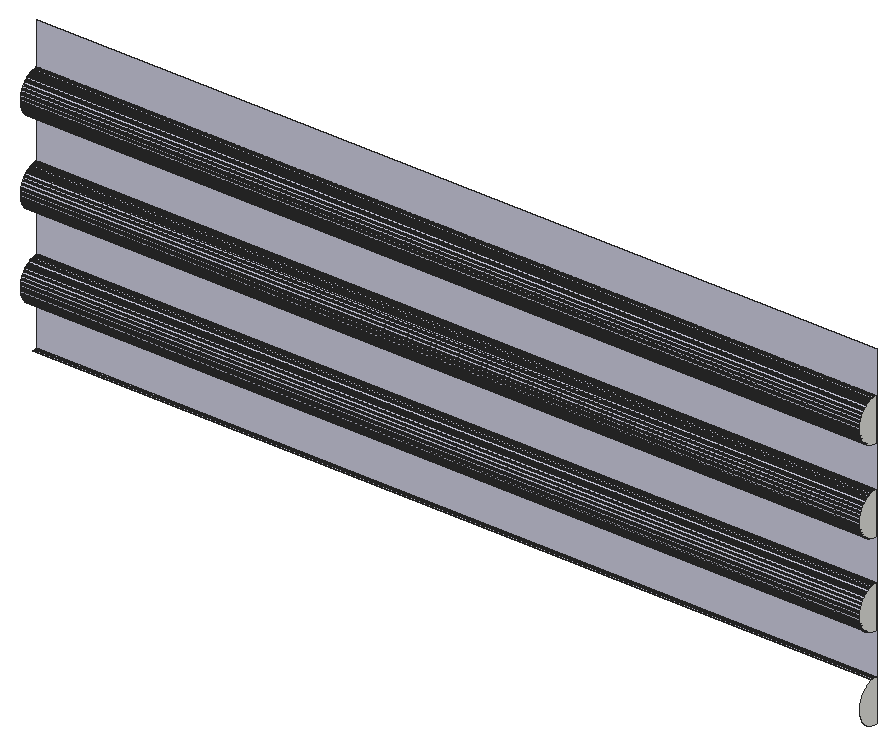
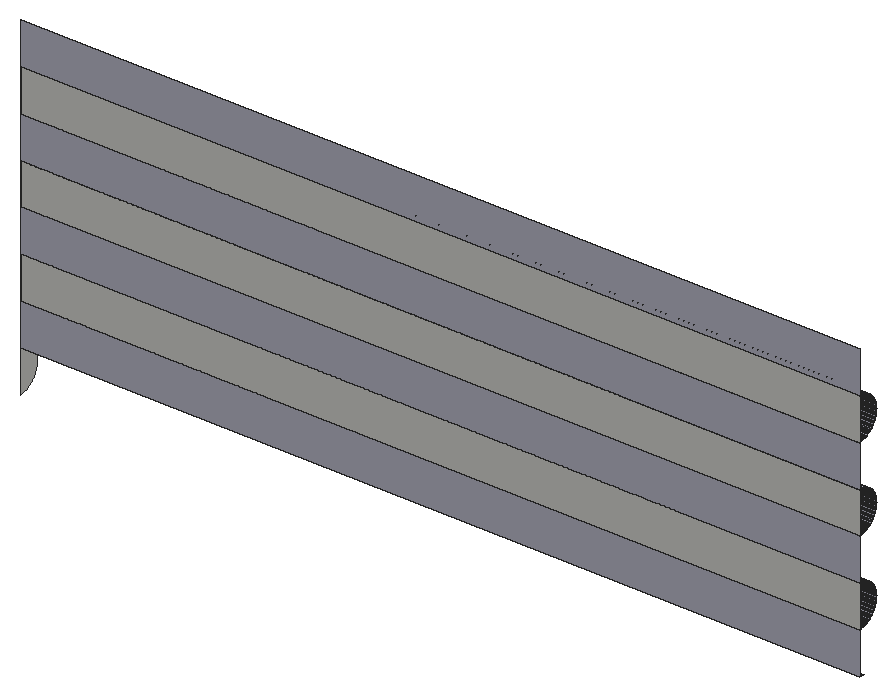
# SketchUp Ruby script. Lengths in millimetres.
U = 1.mm
M = Sketchup.active_model
def pt(a) = Geom::Point3d.new(a.map { |v| v * U })
def face(e, loops, mat)
  f = e.add_face(loops[0].map { |a| pt(a) })
  loops[1..].each { |l| e.add_face(l.map { |a| pt(a) }).erase! }
  f.material = f.back_material = mat if mat
  f
end
# faces: each face lists its corners as indices into pts; further lists are holes
def faces(e, pts, list, mat = nil) = list.each { |f| face(e, (f[0].is_a?(Array) ? f : [f]).map { |l| l.map { |i| pts[i] } }, mat) }
# xy, xz, yz: faces in a plane at the given z, y or x. An outline is a flat list of corners, or four numbers for a rectangle; further outlines are holes
def ring(l) = l.size == 4 ? [[l[0], l[1]], [l[2], l[1]], [l[2], l[3]], [l[0], l[3]]] : l.each_slice(2).to_a
def flat(e, list, mat, &to3) = list.each { |f| face(e, (f[0].is_a?(Array) ? f : [f]).map { |l| ring(l).map { |u, v| to3.(u, v) } }, mat) }
def xy(e, z, list, mat = nil) = flat(e, list, mat) { |x, y| [x, y, z] }
def xz(e, y, list, mat = nil) = flat(e, list, mat) { |x, z| [x, y, z] }
def yz(e, x, list, mat = nil) = flat(e, list, mat) { |y, z| [x, y, z] }
def lines(e, pts, list) = list.each { |a, b| e.add_line(pt(pts[a]), pt(pts[b])) }
# prism: a flat outline (further loops are holes) pulled along v
def prism(e, loops, v, mat = nil)
  f = face(e, loops, mat); d = Geom::Vector3d.new(v.map { |x| x * U })
  f.pushpull(f.normal.samedirection?(d) ? d.length : -d.length)
end
def box(e, o, s, mat = nil) = prism(e, [[o, [o[0] + s[0], o[1], o[2]], [o[0] + s[0], o[1] + s[1], o[2]], [o[0], o[1] + s[1], o[2]]]], [0, 0, s[2]], mat)
def at(x, y, z, deg = 0) = Geom::Transformation.translation(pt([x, y, z])) * Geom::Transformation.rotation(ORIGIN, Z_AXIS, deg.degrees)
def axes(o, x, y, z) = Geom::Transformation.new([*x, 0, *y, 0, *z, 0, *pt(o).to_a, 1])
def part(name) = M.definitions.add(name)
# library, detail: a bought-in or finely detailed component or shape, given as its bounding box
def library(name, o, s) = part(name).tap { |d| box(d.entities, o, s) }
def detail(e, o, s) = box(e.add_group.entities, o, s)
def put(e, d, t, mat = nil) = e.add_instance(d, t).tap { |i| i.material = mat if mat }
def group(e, t, mat = nil) = e.add_group.tap { |g| g.transformation = t; g.material = mat if mat }.entities
root = M.entities
M.materials.add("[0116_Lavender]").color = [197, 197, 214]
xz(root,16548.1,[[29021.7,9312.3,35117.7,9617.1],[29021.7,9921.9,35117.7,10226.7],[29021.7,10531.5,35117.7,10836.3]])
xz(root,16548.1,[[29021.7,9007.5,35117.7,9312.3],[29021.7,9617.1,35117.7,9921.9],[29021.7,10226.7,35117.7,10531.5],[29021.7,10836.3,35117.7,11141.1]],"[0116_Lavender]")
yz(root,35117.7,[[16548.1,8702.7,16548.1,9007.5,16540.1,9007.3,16532.2,9006.6,16524.3,9005.6,16516.4,9004.1,16508.7,9002.3,16501,9000,16493.5,8997.4,16486.1,8994.3,16478.9,8990.9,16471.9,8987.1,16465.1,8982.9,16458.5,8978.4,16452.2,8973.5,16446.1,8968.3,16440.3,8962.8,16434.8,8957.1,16429.7,8951,16424.8,8944.7,16420.3,8938.1,16416.1,8931.3,16412.3,8924.3,16408.9,8917.1,16405.8,8909.7,16403.2,8902.2,16400.9,8894.5,16399,8886.8,16397.6,8878.9,16396.5,8871,16395.9,8863.1,16395.7,8855.1,16395.9,8847.1,16396.5,8839.1,16397.6,8831.2,16399,8823.4,16400.9,8815.6,16403.2,8808,16405.8,8800.5,16408.9,8793.1,16412.3,8785.9,16416.1,8778.9,16420.3,8772.1,16424.8,8765.5,16429.7,8759.2,16434.8,8753.1,16440.3,8747.3,16446.1,8741.8,16452.2,8736.6,16458.5,8731.8,16465.1,8727.3,16471.9,8723.1,16478.9,8719.3,16486.1,8715.9,16493.5,8712.8,16501,8710.1,16508.7,8707.9,16516.4,8706,16524.3,8704.6,16532.2,8703.5,16540.1,8702.9],[16548.1,9312.3,16548.1,9617.1,16540.1,9616.9,16532.2,9616.2,16524.3,9615.2,16516.4,9613.7,16508.7,9611.9,16501,9609.6,16493.5,9607,16486.1,9603.9,16478.9,9600.5,16471.9,9596.7,16465.1,9592.5,16458.5,9588,16452.2,9583.1,16446.1,9577.9,16440.3,9572.4,16434.8,9566.7,16429.7,9560.6,16424.8,9554.3,16420.3,9547.7,16416.1,9540.9,16412.3,9533.9,16408.9,9526.7,16405.8,9519.3,16403.2,9511.8,16400.9,9504.1,16399,9496.4,16397.6,9488.5,16396.5,9480.6,16395.9,9472.7,16395.7,9464.7,16395.9,9456.7,16396.5,9448.7,16397.6,9440.8,16399,9433,16400.9,9425.2,16403.2,9417.6,16405.8,9410.1,16408.9,9402.7,16412.3,9395.5,16416.1,9388.5,16420.3,9381.7,16424.8,9375.1,16429.7,9368.8,16434.8,9362.7,16440.3,9356.9,16446.1,9351.4,16452.2,9346.2,16458.5,9341.4,16465.1,9336.9,16471.9,9332.7,16478.9,9328.9,16486.1,9325.5,16493.5,9322.4,16501,9319.7,16508.7,9317.5,16516.4,9315.6,16524.3,9314.2,16532.2,9313.1,16540.1,9312.5],[16548.1,9921.9,16548.1,10226.7,16540.1,10226.5,16532.2,10225.8,16524.3,10224.8,16516.4,10223.3,16508.7,10221.5,16501,10219.2,16493.5,10216.6,16486.1,10213.5,16478.9,10210.1,16471.9,10206.3,16465.1,10202.1,16458.5,10197.6,16452.2,10192.7,16446.1,10187.5,16440.3,10182,16434.8,10176.3,16429.7,10170.2,16424.8,10163.9,16420.3,10157.3,16416.1,10150.5,16412.3,10143.5,16408.9,10136.3,16405.8,10128.9,16403.2,10121.4,16400.9,10113.7,16399,10106,16397.6,10098.1,16396.5,10090.2,16395.9,10082.3,16395.7,10074.3,16395.9,10066.3,16396.5,10058.3,16397.6,10050.4,16399,10042.6,16400.9,10034.8,16403.2,10027.2,16405.8,10019.7,16408.9,10012.3,16412.3,10005.1,16416.1,9998.1,16420.3,9991.3,16424.8,9984.7,16429.7,9978.4,16434.8,9972.3,16440.3,9966.5,16446.1,9961,16452.2,9955.8,16458.5,9951,16465.1,9946.5,16471.9,9942.3,16478.9,9938.5,16486.1,9935.1,16493.5,9932,16501,9929.3,16508.7,9927.1,16516.4,9925.2,16524.3,9923.8,16532.2,9922.7,16540.1,9922.1],[16548.1,10531.5,16548.1,10836.3,16540.1,10836.1,16532.2,10835.4,16524.3,10834.4,16516.4,10832.9,16508.7,10831.1,16501,10828.8,16493.5,10826.2,16486.1,10823.1,16478.9,10819.7,16471.9,10815.9,16465.1,10811.7,16458.5,10807.2,16452.2,10802.3,16446.1,10797.1,16440.3,10791.6,16434.8,10785.9,16429.7,10779.8,16424.8,10773.5,16420.3,10766.9,16416.1,10760.1,16412.3,10753.1,16408.9,10745.9,16405.8,10738.5,16403.2,10731,16400.9,10723.3,16399,10715.6,16397.6,10707.7,16396.5,10699.8,16395.9,10691.9,16395.7,10683.9,16395.9,10675.9,16396.5,10667.9,16397.6,10660,16399,10652.2,16400.9,10644.4,16403.2,10636.8,16405.8,10629.3,16408.9,10621.9,16412.3,10614.7,16416.1,10607.7,16420.3,10600.9,16424.8,10594.3,16429.7,10588,16434.8,10581.9,16440.3,10576.1,16446.1,10570.6,16452.2,10565.4,16458.5,10560.6,16465.1,10556.1,16471.9,10551.9,16478.9,10548.1,16486.1,10544.7,16493.5,10541.6,16501,10538.9,16508.7,10536.7,16516.4,10534.8,16524.3,10533.4,16532.2,10532.3,16540.1,10531.7]])
p = [[35117.7,16508.7,9002.3],[35117.7,16516.4,9004.1],[29021.7,16516.4,9004.1],[29021.7,16508.7,9002.3],[35117.7,16524.3,9005.6],[29021.7,16524.3,9005.6],
  [35117.7,16532.2,9006.6],[29021.7,16532.2,9006.6],[35117.7,16540.1,9007.3],[29021.7,16540.1,9007.3],[35117.7,16548.1,9007.5],[29021.7,16548.1,9007.5],
  [35117.7,16548.1,9312.3],[35117.7,16540.1,9312.5],[29021.7,16540.1,9312.5],[29021.7,16548.1,9312.3],[35117.7,16532.2,9313.1],[29021.7,16532.2,9313.1],
  [35117.7,16524.3,9314.2],[29021.7,16524.3,9314.2],[35117.7,16516.4,9315.6],[29021.7,16516.4,9315.6],[35117.7,16508.7,9317.5],[29021.7,16508.7,9317.5],
  [35117.7,16501,9319.7],[29021.7,16501,9319.7],[35117.7,16493.5,9322.4],[29021.7,16493.5,9322.4],[35117.7,16486.1,9325.5],[29021.7,16486.1,9325.5],
  [35117.7,16478.9,9328.9],[29021.7,16478.9,9328.9],[35117.7,16471.9,9332.7],[29021.7,16471.9,9332.7],[35117.7,16465.1,9336.9],[29021.7,16465.1,9336.9],
  [35117.7,16458.5,9341.4],[29021.7,16458.5,9341.4],[35117.7,16452.2,9346.2],[29021.7,16452.2,9346.2],[35117.7,16446.1,9351.4],[29021.7,16446.1,9351.4],
  [35117.7,16440.3,9356.9],[29021.7,16440.3,9356.9],[35117.7,16434.8,9362.7],[29021.7,16434.8,9362.7],[35117.7,16429.7,9368.8],[29021.7,16429.7,9368.8],
  [35117.7,16424.8,9375.1],[29021.7,16424.8,9375.1],[35117.7,16420.3,9381.7],[29021.7,16420.3,9381.7],[35117.7,16416.1,9388.5],[29021.7,16416.1,9388.5],
  [35117.7,16412.3,9395.5],[29021.7,16412.3,9395.5],[35117.7,16408.9,9402.7],[29021.7,16408.9,9402.7],[35117.7,16405.8,9410.1],[29021.7,16405.8,9410.1],
  [35117.7,16403.2,9417.6],[29021.7,16403.2,9417.6],[35117.7,16400.9,9425.2],[29021.7,16400.9,9425.2],[35117.7,16399,9433],[29021.7,16399,9433],
  [35117.7,16397.6,9440.8],[29021.7,16397.6,9440.8],[35117.7,16396.5,9448.7],[29021.7,16396.5,9448.7],[35117.7,16395.9,9456.7],[29021.7,16395.9,9456.7],
  [35117.7,16395.7,9464.7],[29021.7,16395.7,9464.7],[35117.7,16395.9,9472.7],[29021.7,16395.9,9472.7],[35117.7,16396.5,9480.6],[29021.7,16396.5,9480.6],
  [35117.7,16397.6,9488.5],[29021.7,16397.6,9488.5],[35117.7,16399,9496.4],[29021.7,16399,9496.4],[35117.7,16400.9,9504.1],[29021.7,16400.9,9504.1],
  [35117.7,16403.2,9511.8],[29021.7,16403.2,9511.8],[35117.7,16405.8,9519.3],[29021.7,16405.8,9519.3],[35117.7,16408.9,9526.7],[29021.7,16408.9,9526.7],
  [35117.7,16412.3,9533.9],[29021.7,16412.3,9533.9],[35117.7,16416.1,9540.9],[29021.7,16416.1,9540.9],[35117.7,16420.3,9547.7],[29021.7,16420.3,9547.7],
  [35117.7,16424.8,9554.3],[29021.7,16424.8,9554.3],[35117.7,16429.7,9560.6],[29021.7,16429.7,9560.6],[35117.7,16434.8,9566.7],[29021.7,16434.8,9566.7],
  [35117.7,16440.3,9572.4],[29021.7,16440.3,9572.4],[35117.7,16446.1,9577.9],[29021.7,16446.1,9577.9],[35117.7,16452.2,9583.1],[29021.7,16452.2,9583.1],
  [35117.7,16458.5,9588],[29021.7,16458.5,9588],[35117.7,16465.1,9592.5],[29021.7,16465.1,9592.5],[35117.7,16471.9,9596.7],[29021.7,16471.9,9596.7],
  [35117.7,16478.9,9600.5],[29021.7,16478.9,9600.5],[35117.7,16486.1,9603.9],[29021.7,16486.1,9603.9],[35117.7,16493.5,9607],[29021.7,16493.5,9607],
  [35117.7,16501,9609.6],[29021.7,16501,9609.6],[35117.7,16508.7,9611.9],[29021.7,16508.7,9611.9],[35117.7,16516.4,9613.7],[29021.7,16516.4,9613.7],
  [35117.7,16524.3,9615.2],[29021.7,16524.3,9615.2],[35117.7,16532.2,9616.2],[29021.7,16532.2,9616.2],[35117.7,16540.1,9616.9],[29021.7,16540.1,9616.9],
  [35117.7,16548.1,9617.1],[29021.7,16548.1,9617.1],[35117.7,16548.1,9921.9],[35117.7,16540.1,9922.1],[29021.7,16540.1,9922.1],[29021.7,16548.1,9921.9],
  [35117.7,16532.2,9922.7],[29021.7,16532.2,9922.7],[35117.7,16524.3,9923.8],[29021.7,16524.3,9923.8],[35117.7,16516.4,9925.2],[29021.7,16516.4,9925.2],
  [35117.7,16508.7,9927.1],[29021.7,16508.7,9927.1],[35117.7,16501,9929.3],[29021.7,16501,9929.3],[35117.7,16493.5,9932],[29021.7,16493.5,9932],
  [35117.7,16486.1,9935.1],[29021.7,16486.1,9935.1],[35117.7,16478.9,9938.5],[29021.7,16478.9,9938.5],[35117.7,16471.9,9942.3],[29021.7,16471.9,9942.3],
  [35117.7,16465.1,9946.5],[29021.7,16465.1,9946.5],[35117.7,16458.5,9951],[29021.7,16458.5,9951],[35117.7,16452.2,9955.8],[29021.7,16452.2,9955.8],
  [35117.7,16446.1,9961],[29021.7,16446.1,9961],[35117.7,16440.3,9966.5],[29021.7,16440.3,9966.5],[35117.7,16434.8,9972.3],[29021.7,16434.8,9972.3],
  [35117.7,16429.7,9978.4],[29021.7,16429.7,9978.4],[35117.7,16424.8,9984.7],[29021.7,16424.8,9984.7],[35117.7,16420.3,9991.3],[29021.7,16420.3,9991.3],
  [35117.7,16416.1,9998.1],[29021.7,16416.1,9998.1],[35117.7,16412.3,10005.1],[29021.7,16412.3,10005.1],[35117.7,16408.9,10012.3],[29021.7,16408.9,10012.3],
  [35117.7,16405.8,10019.7],[29021.7,16405.8,10019.7],[35117.7,16403.2,10027.2],[29021.7,16403.2,10027.2],[35117.7,16400.9,10034.8],[29021.7,16400.9,10034.8],
  [35117.7,16399,10042.6],[29021.7,16399,10042.6],[35117.7,16397.6,10050.4],[29021.7,16397.6,10050.4],[35117.7,16396.5,10058.3],[29021.7,16396.5,10058.3],
  [35117.7,16395.9,10066.3],[29021.7,16395.9,10066.3],[35117.7,16395.7,10074.3],[29021.7,16395.7,10074.3],[35117.7,16395.9,10082.3],[29021.7,16395.9,10082.3],
  [35117.7,16396.5,10090.2],[29021.7,16396.5,10090.2],[35117.7,16397.6,10098.1],[29021.7,16397.6,10098.1],[35117.7,16399,10106],[29021.7,16399,10106],
  [35117.7,16400.9,10113.7],[29021.7,16400.9,10113.7],[35117.7,16403.2,10121.4],[29021.7,16403.2,10121.4],[35117.7,16405.8,10128.9],[29021.7,16405.8,10128.9],
  [35117.7,16408.9,10136.3],[29021.7,16408.9,10136.3],[35117.7,16412.3,10143.5],[29021.7,16412.3,10143.5],[35117.7,16416.1,10150.5],[29021.7,16416.1,10150.5],
  [35117.7,16420.3,10157.3],[29021.7,16420.3,10157.3],[35117.7,16424.8,10163.9],[29021.7,16424.8,10163.9],[35117.7,16429.7,10170.2],[29021.7,16429.7,10170.2],
  [35117.7,16434.8,10176.3],[29021.7,16434.8,10176.3],[35117.7,16440.3,10182],[29021.7,16440.3,10182],[35117.7,16446.1,10187.5],[29021.7,16446.1,10187.5],
  [35117.7,16452.2,10192.7],[29021.7,16452.2,10192.7],[35117.7,16458.5,10197.6],[29021.7,16458.5,10197.6],[35117.7,16465.1,10202.1],[29021.7,16465.1,10202.1],
  [35117.7,16471.9,10206.3],[29021.7,16471.9,10206.3],[35117.7,16478.9,10210.1],[29021.7,16478.9,10210.1],[35117.7,16486.1,10213.5],[29021.7,16486.1,10213.5],
  [35117.7,16493.5,10216.6],[29021.7,16493.5,10216.6],[35117.7,16501,10219.2],[29021.7,16501,10219.2],[35117.7,16508.7,10221.5],[29021.7,16508.7,10221.5],
  [35117.7,16516.4,10223.3],[29021.7,16516.4,10223.3],[35117.7,16524.3,10224.8],[29021.7,16524.3,10224.8],[35117.7,16532.2,10225.8],[29021.7,16532.2,10225.8],
  [35117.7,16540.1,10226.5],[29021.7,16540.1,10226.5],[35117.7,16548.1,10226.7],[29021.7,16548.1,10226.7],[35117.7,16548.1,10531.5],[35117.7,16540.1,10531.7],
  [29021.7,16540.1,10531.7],[29021.7,16548.1,10531.5],[35117.7,16532.2,10532.3],[29021.7,16532.2,10532.3],[35117.7,16524.3,10533.4],[29021.7,16524.3,10533.4],
  [35117.7,16516.4,10534.8],[29021.7,16516.4,10534.8],[35117.7,16508.7,10536.7],[29021.7,16508.7,10536.7],[35117.7,16501,10538.9],[29021.7,16501,10538.9],
  [35117.7,16493.5,10541.6],[29021.7,16493.5,10541.6],[35117.7,16486.1,10544.7],[29021.7,16486.1,10544.7],[35117.7,16478.9,10548.1],[29021.7,16478.9,10548.1],
  [35117.7,16471.9,10551.9],[29021.7,16471.9,10551.9],[35117.7,16465.1,10556.1],[29021.7,16465.1,10556.1],[35117.7,16458.5,10560.6],[29021.7,16458.5,10560.6],
  [35117.7,16452.2,10565.4],[29021.7,16452.2,10565.4],[35117.7,16446.1,10570.6],[29021.7,16446.1,10570.6],[35117.7,16440.3,10576.1],[29021.7,16440.3,10576.1],
  [35117.7,16434.8,10581.9],[29021.7,16434.8,10581.9],[35117.7,16429.7,10588],[29021.7,16429.7,10588],[35117.7,16424.8,10594.3],[29021.7,16424.8,10594.3],
  [35117.7,16420.3,10600.9],[29021.7,16420.3,10600.9],[35117.7,16416.1,10607.7],[29021.7,16416.1,10607.7],[35117.7,16412.3,10614.7],[29021.7,16412.3,10614.7],
  [35117.7,16408.9,10621.9],[29021.7,16408.9,10621.9],[35117.7,16405.8,10629.3],[29021.7,16405.8,10629.3],[35117.7,16403.2,10636.8],[29021.7,16403.2,10636.8],
  [35117.7,16400.9,10644.4],[29021.7,16400.9,10644.4],[35117.7,16399,10652.2],[29021.7,16399,10652.2],[35117.7,16397.6,10660],[29021.7,16397.6,10660],
  [35117.7,16396.5,10667.9],[29021.7,16396.5,10667.9],[35117.7,16395.9,10675.9],[29021.7,16395.9,10675.9],[35117.7,16395.7,10683.9],[29021.7,16395.7,10683.9],
  [35117.7,16395.9,10691.9],[29021.7,16395.9,10691.9],[35117.7,16396.5,10699.8],[29021.7,16396.5,10699.8],[35117.7,16397.6,10707.7],[29021.7,16397.6,10707.7],
  [35117.7,16399,10715.6],[29021.7,16399,10715.6],[35117.7,16400.9,10723.3],[29021.7,16400.9,10723.3],[35117.7,16403.2,10731],[29021.7,16403.2,10731],
  [35117.7,16405.8,10738.5],[29021.7,16405.8,10738.5],[35117.7,16408.9,10745.9],[29021.7,16408.9,10745.9],[35117.7,16412.3,10753.1],[29021.7,16412.3,10753.1],
  [35117.7,16416.1,10760.1],[29021.7,16416.1,10760.1],[35117.7,16420.3,10766.9],[29021.7,16420.3,10766.9],[35117.7,16424.8,10773.5],[29021.7,16424.8,10773.5],
  [35117.7,16429.7,10779.8],[29021.7,16429.7,10779.8],[35117.7,16434.8,10785.9],[29021.7,16434.8,10785.9],[35117.7,16440.3,10791.6],[29021.7,16440.3,10791.6],
  [35117.7,16446.1,10797.1],[29021.7,16446.1,10797.1],[35117.7,16452.2,10802.3],[29021.7,16452.2,10802.3],[35117.7,16458.5,10807.2],[29021.7,16458.5,10807.2],
  [35117.7,16465.1,10811.7],[29021.7,16465.1,10811.7],[35117.7,16471.9,10815.9],[29021.7,16471.9,10815.9],[35117.7,16478.9,10819.7],[29021.7,16478.9,10819.7],
  [35117.7,16486.1,10823.1],[29021.7,16486.1,10823.1],[35117.7,16493.5,10826.2],[29021.7,16493.5,10826.2],[35117.7,16501,10828.8],[29021.7,16501,10828.8],
  [35117.7,16508.7,10831.1],[29021.7,16508.7,10831.1],[35117.7,16516.4,10832.9],[29021.7,16516.4,10832.9],[35117.7,16524.3,10834.4],[29021.7,16524.3,10834.4],
  [35117.7,16532.2,10835.4],[29021.7,16532.2,10835.4],[35117.7,16540.1,10836.1],[29021.7,16540.1,10836.1],[35117.7,16548.1,10836.3],[29021.7,16548.1,10836.3]]
faces(root,p,[[0,1,2,3],[1,4,5,2],[4,6,7,5],[6,8,9,7],[8,10,11,9],[12,13,14,15],[13,16,17,14],[16,18,19,17],
  [18,20,21,19],[20,22,23,21],[22,24,25,23],[24,26,27,25],[26,28,29,27],[28,30,31,29],[30,32,33,31],[32,34,35,33],
  [34,36,37,35],[36,38,39,37],[38,40,41,39],[40,42,43,41],[42,44,45,43],[44,46,47,45],[46,48,49,47],[48,50,51,49],
  [50,52,53,51],[52,54,55,53],[54,56,57,55],[56,58,59,57],[58,60,61,59],[60,62,63,61],[62,64,65,63],[64,66,67,65],
  [66,68,69,67],[68,70,71,69],[70,72,73,71],[72,74,75,73],[74,76,77,75],[76,78,79,77],[78,80,81,79],[80,82,83,81],
  [82,84,85,83],[84,86,87,85],[86,88,89,87],[88,90,91,89],[90,92,93,91],[92,94,95,93],[94,96,97,95],[96,98,99,97],
  [98,100,101,99],[100,102,103,101],[102,104,105,103],[104,106,107,105],[106,108,109,107],[108,110,111,109],[110,112,113,111],[112,114,115,113],
  [114,116,117,115],[116,118,119,117],[118,120,121,119],[120,122,123,121],[122,124,125,123],[124,126,127,125],[126,128,129,127],[128,130,131,129],
  [130,132,133,131],[134,135,136,137],[135,138,139,136],[138,140,141,139],[140,142,143,141],[142,144,145,143],[144,146,147,145],[146,148,149,147],
  [148,150,151,149],[150,152,153,151],[152,154,155,153],[154,156,157,155],[156,158,159,157],[158,160,161,159],[160,162,163,161],[162,164,165,163],
  [164,166,167,165],[166,168,169,167],[168,170,171,169],[170,172,173,171],[172,174,175,173],[174,176,177,175],[176,178,179,177],[178,180,181,179],
  [180,182,183,181],[182,184,185,183],[184,186,187,185],[186,188,189,187],[188,190,191,189],[190,192,193,191],[192,194,195,193],[194,196,197,195],
  [196,198,199,197],[198,200,201,199],[200,202,203,201],[202,204,205,203],[204,206,207,205],[206,208,209,207],[208,210,211,209],[210,212,213,211],
  [212,214,215,213],[214,216,217,215],[216,218,219,217],[218,220,221,219],[220,222,223,221],[222,224,225,223],[224,226,227,225],[226,228,229,227],
  [228,230,231,229],[230,232,233,231],[232,234,235,233],[234,236,237,235],[236,238,239,237],[238,240,241,239],[240,242,243,241],[242,244,245,243],
  [244,246,247,245],[246,248,249,247],[248,250,251,249],[250,252,253,251],[252,254,255,253],[256,257,258,259],[257,260,261,258],[260,262,263,261],
  [262,264,265,263],[264,266,267,265],[266,268,269,267],[268,270,271,269],[270,272,273,271],[272,274,275,273],[274,276,277,275],[276,278,279,277],
  [278,280,281,279],[280,282,283,281],[282,284,285,283],[284,286,287,285],[286,288,289,287],[288,290,291,289],[290,292,293,291],[292,294,295,293],
  [294,296,297,295],[296,298,299,297],[298,300,301,299],[300,302,303,301],[302,304,305,303],[304,306,307,305],[306,308,309,307],[308,310,311,309],
  [310,312,313,311],[312,314,315,313],[314,316,317,315],[316,318,319,317],[318,320,321,319],[320,322,323,321],[322,324,325,323],[324,326,327,325],
  [326,328,329,327],[328,330,331,329],[330,332,333,331],[332,334,335,333],[334,336,337,335],[336,338,339,337],[338,340,341,339],[340,342,343,341],
  [342,344,345,343],[344,346,347,345],[346,348,349,347],[348,350,351,349],[350,352,353,351],[352,354,355,353],[354,356,357,355],[356,358,359,357],
  [358,360,361,359],[360,362,363,361],[362,364,365,363],[364,366,367,365],[366,368,369,367],[368,370,371,369],[370,372,373,371],[372,374,375,373],
  [374,376,377,375]],"[0116_Lavender]")
